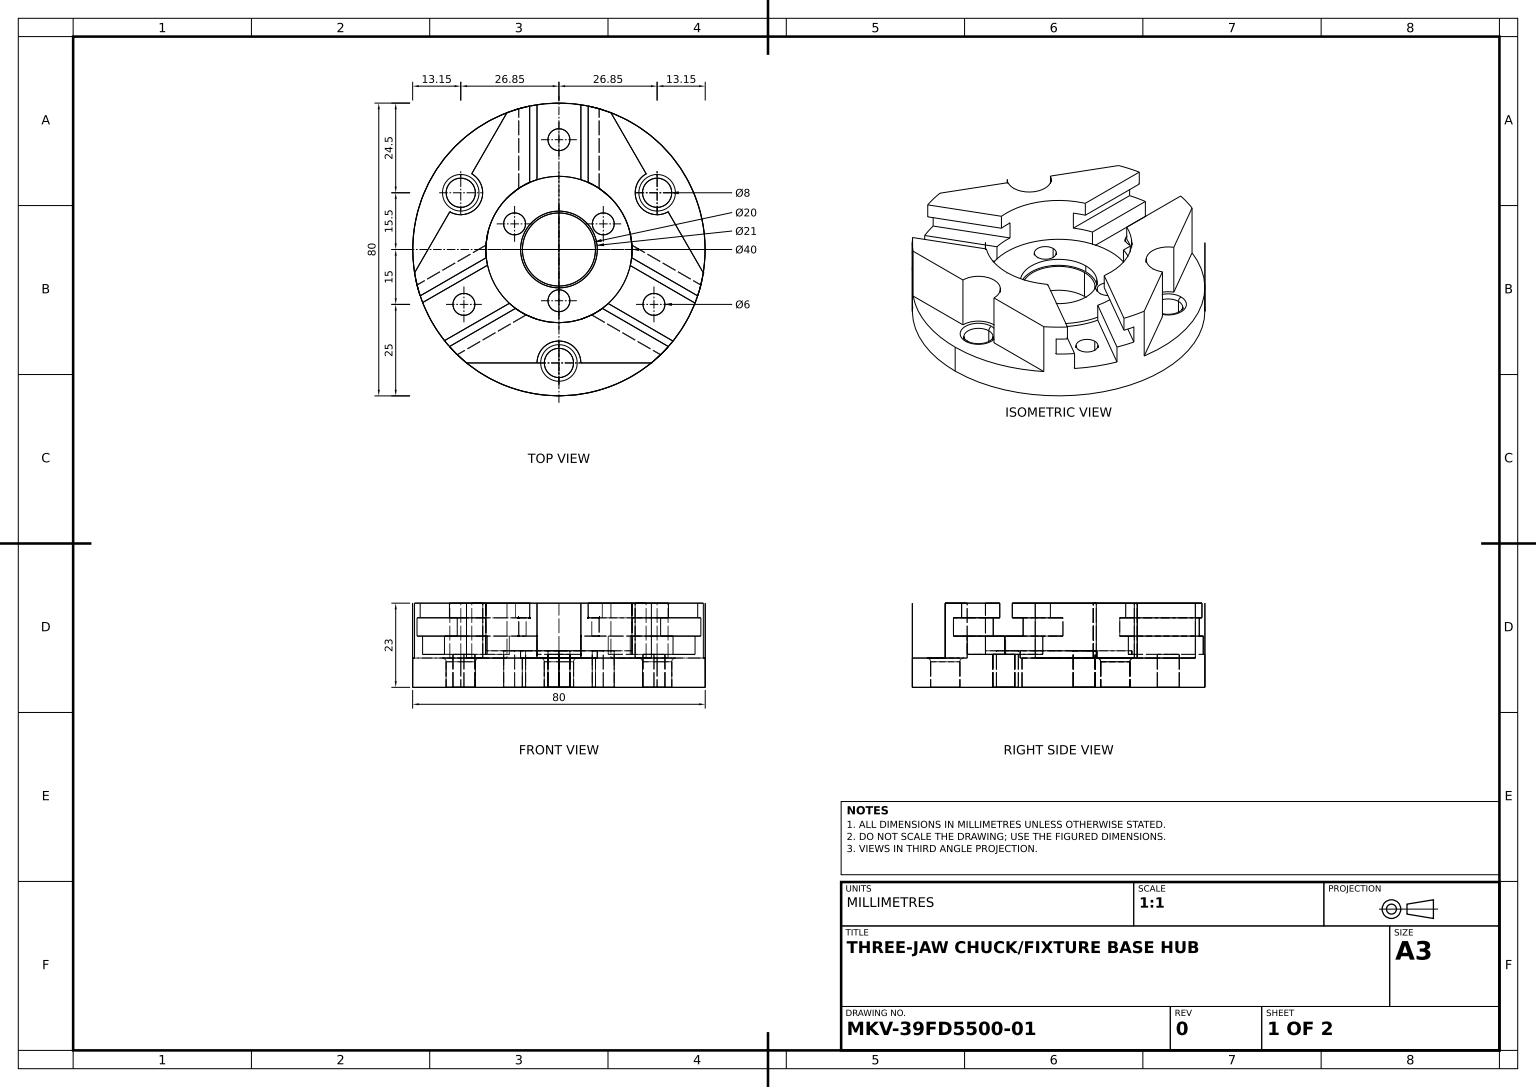
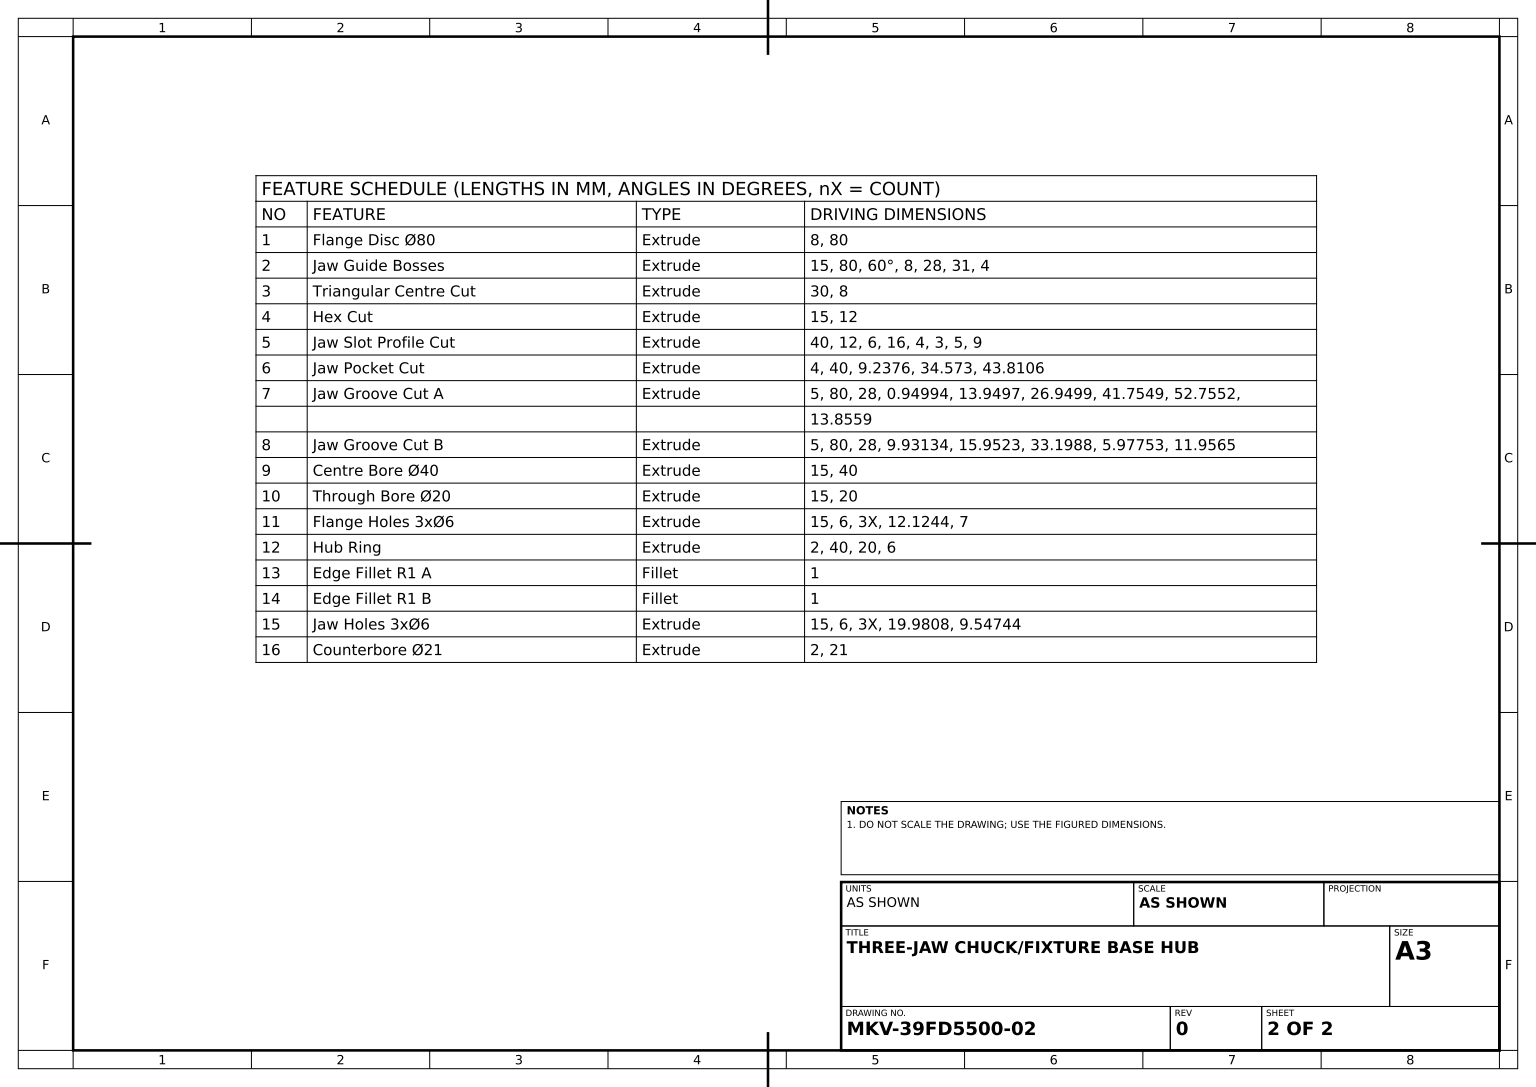
solid
v1 (25.980762,0,18)
v2 (25.980762,9,18)
e1 v1 v2 LINE
v3 (25.980762,9,12)
e2 v2 v3 CIRCLE(AX(P(25.980762,9,15),D(0,1,0),D(0,0,1)),3)
v4 (25.980762,0,12)
e3 v4 v3 LINE
e4 v1 v4 CIRCLE(AX(P(25.980762,0,15),D(0,1,0),D(0,0,1)),3)
face CYL(AX(P(25.980762,-6,15),D(0,1,0),D(0,0,1)),3) rev [e1 e2 -e3 -e4]
v5 (0,0,-10)
v6 (0,8,-10)
e5 v5 v6 LINE
v7 (0,8,10)
e6 v7 v6 CIRCLE(AX(P(0,8,0),D(0,-1,0),D(0,0,1)),10)
v8 (0,0,10)
e7 v8 v7 LINE
e8 v5 v8 CIRCLE(AX(P(0,0,0),D(0,1,0),D(0,0,1)),10)
face CYL(AX(P(0,-7,0),D(0,1,0),D(0,0,1)),10) rev [e5 -e6 -e7 -e8]
v9 (29.846788,8,-10.303848)
v10 (29.846788,23,-10.303848)
e9 v9 v10 LINE
v11 (26.846788,8,-9.5)
e10 v11 v9 CIRCLE(AX(P(26.846788,8,-15.5),D(0,1,0),D(0,0,1)),6)
v12 (26.846788,23,-9.5)
e11 v11 v12 LINE
e12 v12 v10 CIRCLE(AX(P(26.846788,23,-15.5),D(0,1,0),D(0,0,1)),6)
face CYL(AX(P(26.846788,8,-15.5),D(0,1,0),D(0,0,1)),6) rev [-e9 -e10 e11 e12]
v13 (-12.124356,0,-10)
v14 (-12.124356,0,-4)
e13 v13 v14 CIRCLE(AX(P(-12.124356,0,-7),D(0,1,0),D(0,0,1)),3)
v15 (-12.124356,10,-10)
e14 v13 v15 LINE
v16 (-12.124356,10,-4)
e15 v15 v16 CIRCLE(AX(P(-12.124356,10,-7),D(0,1,0),D(0,0,1)),3)
e16 v14 v16 LINE
face CYL(AX(P(-12.124356,-7,-7),D(0,1,0),D(0,0,1)),3) rev [-e13 e14 e15 -e16]
v17 (-8.965703,14,17.877812)
v18 (-27.80577,14,28.754811)
e17 v17 v18 LINE
v19 (-27.80577,19,28.754811)
e18 v18 v19 LINE
v20 (-8.965703,19,17.877812)
e19 v20 v19 LINE
e20 v17 v20 LINE
face PLANE(AX(P(5.499879,14,9.526349),D(-0.499989,0,-0.866031755),D(-0.866031755,0,0.499989))) [e17 e18 -e19 -e20]
v21 (-13.552446,9,14.708202)
v22 (-13.552446,10,14.708202)
e21 v21 v22 LINE
v23 (-19.531444,10,4.3038)
e22 v23 v22 CIRCLE(AX(P(0,10,0),D(0,1,0),D(0,0,1)),20)
v24 (-19.531444,9,4.3038)
e23 v24 v23 LINE
e24 v24 v21 CIRCLE(AX(P(0,9,0),D(0,1,0),D(0,0,1)),20)
face CYL(AX(P(0,10,0),D(0,-1,0),D(0,0,-1)),20) [e21 -e22 -e23 e24]
v25 (-26.846788,0,-11.5)
v26 (-26.846788,0,-19.5)
e25 v25 v26 CIRCLE(AX(P(-26.846788,0,-15.5),D(0,1,0),D(0,0,1)),4)
v27 (-26.846788,7,-11.5)
e26 v27 v25 LINE
v28 (-26.846788,7,-19.5)
e27 v27 v28 CIRCLE(AX(P(-26.846788,7,-15.5),D(0,1,0),D(0,0,1)),4)
e28 v28 v26 LINE
face CYL(AX(P(-26.846788,23,-15.5),D(0,-1,0),D(0,0,-1)),4) rev [-e25 -e26 e27 e28]
e29 v3 v2 CIRCLE(AX(P(25.980762,9,15),D(0,1,0),D(0,0,1)),3)
v29 (31.198591,9,25.032936)
v30 (37.219569,9,14.652771)
e30 v29 v30 CIRCLE(AX(P(0,9,0),D(0,1,0),D(0,0,1)),40)
v31 (19.5139,9,4.382662)
e31 v30 v31 LINE
v32 (13.492922,9,14.762827)
e32 v32 v31 CIRCLE(AX(P(0,9,0),D(0,1,0),D(0,0,1)),20)
e33 v32 v29 LINE
face PLANE(AX(P(0,9,0),D(0,1,0),D(0,0,1))) [-e2 -e29] [e30 e31 -e32 e33]
v33 (-8,19,-18.330303)
v34 (-8,19,-39.191836)
e34 v33 v34 LINE
v35 (-11,19,-16.703293)
e35 v35 v33 CIRCLE(AX(P(0,19,0),D(0,-1,0),D(0,0,-1)),20)
v36 (-11,19,-38.457769)
e36 v35 v36 LINE
e37 v36 v34 CIRCLE(AX(P(0,19,0),D(0,-1,0),D(0,0,-1)),40)
face PLANE(AX(P(-8,19,0),D(0,-1,0),D(0,0,-1))) [-e34 -e35 e36 e37]
v37 (8,23,-18.330303)
v38 (8,19,-18.330303)
e38 v37 v38 LINE
v39 (11,19,-16.703293)
e39 v38 v39 CIRCLE(AX(P(0,19,0),D(0,-1,0),D(0,0,-1)),20)
v40 (11,14,-16.703293)
e40 v39 v40 LINE
v41 (6,14,-19.078784)
e41 v40 v41 CIRCLE(AX(P(0,14,0),D(0,1,0),D(-1,0,0)),20)
v42 (6,10,-19.078784)
e42 v41 v42 LINE
v43 (19.5139,10,4.382662)
e43 v43 v42 CIRCLE(AX(P(0,10,0),D(0,1,0),D(0,0,1)),20)
v44 (19.5139,14,4.382662)
e44 v44 v43 LINE
v45 (19.965491,14,-1.174379)
e45 v44 v45 CIRCLE(AX(P(0,14,0),D(0,1,0),D(0,0,1)),20)
v46 (19.965491,19,-1.174379)
e46 v45 v46 LINE
v47 (19.874508,19,2.236948)
e47 v47 v46 CIRCLE(AX(P(0,19,0),D(0,1,0),D(0,0,1)),20)
v48 (19.874508,23,2.236948)
e48 v48 v47 LINE
e49 v48 v37 CIRCLE(AX(P(0,23,0),D(0,1,0),D(0,0,1)),20)
face CYL(AX(P(0,8,0),D(0,1,0),D(0,0,1)),20) rev [e38 e39 e40 e41 e42 -e43 -e44 e45 e46 -e47 -e48 e49]
v49 (13.492922,10,14.762827)
v50 (13.492922,14,14.762827)
e50 v49 v50 LINE
v51 (31.198591,14,25.032936)
e51 v50 v51 LINE
e52 v29 v51 LINE
e53 v32 v49 LINE
face PLANE(AX(P(7.931166,9,11.53675),D(-0.501748125,0,0.865013768),D(0.865013768,0,0.501748125))) rev [e50 e51 -e52 -e33 e53]
v52 (-37.278454,9,14.502304)
e54 v24 v52 LINE
v53 (-31.299456,9,24.906706)
e55 v52 v53 CIRCLE(AX(P(0,9,0),D(0,1,0),D(0,0,1)),40)
e56 v53 v21 LINE
v54 (-25.980762,9,18)
v55 (-25.980762,9,12)
e57 v54 v55 CIRCLE(AX(P(-25.980762,9,15),D(0,1,0),D(0,0,1)),3)
e58 v55 v54 CIRCLE(AX(P(-25.980762,9,15),D(0,1,0),D(0,0,1)),3)
face PLANE(AX(P(0,9,0),D(0,1,0),D(0,0,1))) [-e24 e54 e55 e56] [-e57 -e58]
v56 (14.207563,23,-37.391779)
v57 (8,23,-39.191836)
e59 v56 v57 CIRCLE(AX(P(0,23,0),D(0,1,0),D(0,0,1)),40)
v58 (14.207563,8,-37.391779)
e60 v56 v58 LINE
v59 (39.486012,8,6.391779)
e61 v59 v58 CIRCLE(AX(P(0,8,0),D(0,1,0),D(0,0,1)),40)
v60 (39.486012,23,6.391779)
e62 v60 v59 LINE
v61 (37.941125,23,12.667715)
e63 v61 v60 CIRCLE(AX(P(0,23,0),D(0,1,0),D(0,0,1)),40)
v62 (37.941125,19,12.667715)
e64 v62 v61 LINE
v63 (38.805282,19,9.703098)
e65 v62 v63 CIRCLE(AX(P(0,19,0),D(0,1,0),D(0,0,1)),40)
v64 (38.805282,14,9.703098)
e66 v64 v63 LINE
v65 (37.219569,14,14.652771)
e67 v65 v64 CIRCLE(AX(P(0,14,0),D(0,1,0),D(0,0,1)),40)
e68 v30 v65 LINE
v66 (27.80504,14,28.755517)
e69 v66 v51 CIRCLE(AX(P(0,14,0),D(0,1,0),D(0,0,1)),40)
v67 (27.80504,19,28.755517)
e70 v66 v67 LINE
v68 (29.941125,19,26.524121)
e71 v67 v68 CIRCLE(AX(P(0,19,0),D(0,1,0),D(0,0,1)),40)
v69 (29.941125,23,26.524121)
e72 v68 v69 LINE
v70 (25.278449,23,31)
e73 v70 v69 CIRCLE(AX(P(0,23,0),D(0,1,0),D(0,0,1)),40)
v71 (25.278449,8,31)
e74 v70 v71 LINE
v72 (0,8,40)
e75 v72 v71 CIRCLE(AX(P(0,8,0),D(0,1,0),D(0,0,1)),40)
v73 (0,0,40)
e76 v72 v73 LINE
v74 (0,0,-40)
e77 v73 v74 CIRCLE(AX(P(0,0,0),D(0,1,0),D(0,0,1)),40)
v75 (0,9,-40)
e78 v75 v74 LINE
v76 (6,9,-39.54744)
e79 v76 v75 CIRCLE(AX(P(0,9,0),D(0,1,0),D(0,0,1)),40)
v77 (6,14,-39.54744)
e80 v77 v76 LINE
v78 (11,14,-38.457769)
e81 v78 v77 CIRCLE(AX(P(0,14,0),D(0,1,0),D(-1,0,0)),40)
v79 (11,19,-38.457769)
e82 v79 v78 LINE
v80 (8,19,-39.191836)
e83 v80 v79 CIRCLE(AX(P(0,19,0),D(0,-1,0),D(0,0,-1)),40)
e84 v57 v80 LINE
face CYL(AX(P(0,8,0),D(0,-1,0),D(0,0,-1)),40) [-e59 e60 -e61 -e62 -e63 -e64 e65 -e66 -e67 -e68 -e30 e52 -e69 e70 e71 e72 -e73 e74 -e75 e76 e77 -e78 -e79 -e80 -e81 -e82 -e83 -e84]
v81 (-25.980762,0,12)
e85 v81 v55 LINE
v82 (-25.980762,0,18)
e86 v82 v81 CIRCLE(AX(P(-25.980762,0,15),D(0,1,0),D(0,0,1)),3)
e87 v82 v54 LINE
face CYL(AX(P(-25.980762,-6,15),D(0,1,0),D(0,0,1)),3) rev [e57 -e85 -e86 e87]
v83 (12.124356,0,-4)
v84 (12.124356,0,-10)
e88 v83 v84 CIRCLE(AX(P(12.124356,0,-7),D(0,1,0),D(0,0,1)),3)
v85 (12.124356,10,-4)
e89 v83 v85 LINE
v86 (12.124356,10,-10)
e90 v85 v86 CIRCLE(AX(P(12.124356,10,-7),D(0,1,0),D(0,0,1)),3)
e91 v84 v86 LINE
face CYL(AX(P(12.124356,-7,-7),D(0,1,0),D(0,0,1)),3) rev [-e88 e89 e90 -e91]
v87 (-8,23,-18.330303)
e92 v33 v87 LINE
v88 (-19.874508,23,2.236948)
e93 v87 v88 CIRCLE(AX(P(0,23,0),D(0,1,0),D(0,0,1)),20)
v89 (-19.874508,19,2.236948)
e94 v89 v88 LINE
v90 (-19.965461,19,-1.174887)
e95 v90 v89 CIRCLE(AX(P(0,19,0),D(0,1,0),D(0,0,1)),20)
v91 (-19.965461,14,-1.174887)
e96 v91 v90 LINE
v92 (-19.531444,14,4.3038)
e97 v91 v92 CIRCLE(AX(P(0,14,0),D(0,1,0),D(0,0,1)),20)
e98 v23 v92 LINE
v93 (-6,10,-19.078784)
e99 v93 v23 CIRCLE(AX(P(0,10,0),D(0,1,0),D(0,0,1)),20)
v94 (-6,14,-19.078784)
e100 v93 v94 LINE
v95 (-11,14,-16.703293)
e101 v94 v95 CIRCLE(AX(P(0,14,0),D(0,1,0),D(0,0,1)),20)
e102 v95 v35 LINE
face CYL(AX(P(0,8,0),D(0,1,0),D(0,0,1)),20) rev [e92 e93 -e94 -e95 -e96 e97 -e98 -e99 e100 e101 e102 e35]
v96 (26.846788,0,-19.5)
v97 (26.846788,0,-11.5)
e103 v96 v97 CIRCLE(AX(P(26.846788,0,-15.5),D(0,1,0),D(0,0,1)),4)
v98 (26.846788,7,-19.5)
e104 v98 v96 LINE
v99 (26.846788,7,-11.5)
e105 v98 v99 CIRCLE(AX(P(26.846788,7,-15.5),D(0,1,0),D(0,0,1)),4)
e106 v99 v97 LINE
face CYL(AX(P(26.846788,23,-15.5),D(0,-1,0),D(0,0,-1)),4) rev [-e103 -e104 e105 e106]
v100 (-6,9,-39.54744)
e107 v75 v100 CIRCLE(AX(P(0,9,0),D(0,1,0),D(0,0,1)),40)
e108 v74 v73 CIRCLE(AX(P(0,0,0),D(0,1,0),D(0,0,1)),40)
v101 (-25.278449,8,31)
e109 v101 v72 CIRCLE(AX(P(0,8,0),D(0,1,0),D(0,0,1)),40)
v102 (-25.278449,23,31)
e110 v102 v101 LINE
v103 (-29.941125,23,26.524121)
e111 v103 v102 CIRCLE(AX(P(0,23,0),D(0,1,0),D(0,0,1)),40)
v104 (-29.941125,19,26.524121)
e112 v104 v103 LINE
e113 v104 v19 CIRCLE(AX(P(0,19,0),D(0,1,0),D(0,0,1)),40)
v105 (-31.299456,14,24.906706)
e114 v105 v18 CIRCLE(AX(P(0,14,0),D(0,1,0),D(0,0,1)),40)
e115 v53 v105 LINE
v106 (-37.278454,14,14.502304)
e116 v52 v106 LINE
v107 (-38.805528,14,9.702112)
e117 v107 v106 CIRCLE(AX(P(0,14,0),D(0,1,0),D(0,0,1)),40)
v108 (-38.805528,19,9.702112)
e118 v107 v108 LINE
v109 (-37.941125,19,12.667715)
e119 v108 v109 CIRCLE(AX(P(0,19,0),D(0,1,0),D(0,0,1)),40)
v110 (-37.941125,23,12.667715)
e120 v109 v110 LINE
v111 (-39.486012,23,6.391779)
e121 v111 v110 CIRCLE(AX(P(0,23,0),D(0,1,0),D(0,0,1)),40)
v112 (-39.486012,8,6.391779)
e122 v111 v112 LINE
v113 (-14.207563,8,-37.391779)
e123 v113 v112 CIRCLE(AX(P(0,8,0),D(0,1,0),D(0,0,1)),40)
v114 (-14.207563,23,-37.391779)
e124 v114 v113 LINE
v115 (-8,23,-39.191836)
e125 v115 v114 CIRCLE(AX(P(0,23,0),D(0,1,0),D(0,0,1)),40)
e126 v34 v115 LINE
v116 (-11,14,-38.457769)
e127 v116 v36 LINE
v117 (-6,14,-39.54744)
e128 v117 v116 CIRCLE(AX(P(0,14,0),D(0,1,0),D(0,0,1)),40)
e129 v100 v117 LINE
face CYL(AX(P(0,8,0),D(0,-1,0),D(0,0,-1)),40) [-e107 e78 e108 -e76 -e109 -e110 -e111 -e112 e113 -e18 -e114 -e115 -e55 e116 -e117 e118 e119 e120 -e121 e122 -e123 -e124 -e125 -e126 -e37 -e127 -e128 -e129]
e130 v87 v115 LINE
v118 (-23.846788,23,-20.696152)
e131 v114 v118 LINE
v119 (-26.846788,23,-9.5)
e132 v119 v118 CIRCLE(AX(P(-26.846788,23,-15.5),D(0,1,0),D(0,0,1)),6)
v120 (-29.846788,23,-10.303848)
e133 v120 v119 CIRCLE(AX(P(-26.846788,23,-15.5),D(0,1,0),D(0,0,1)),6)
e134 v120 v111 LINE
e135 v88 v110 LINE
face PLANE(AX(P(0,23,0),D(0,1,0),D(0,0,1))) [e130 e125 e131 -e132 -e133 e134 e121 -e135 -e93]
e136 v39 v79 LINE
e137 v40 v78 LINE
face PLANE(AX(P(11,19,0),D(-1,0,0),D(0,-1,0))) [e136 e82 -e137 -e40]
v121 (6,8,31)
v122 (-6,8,31)
e138 v121 v122 CIRCLE(AX(P(0,8,31),D(0,1,0),D(0,0,1)),6)
e139 v122 v101 LINE
e140 v71 v121 LINE
v123 (0,8,36)
v124 (0,8,26)
e141 v123 v124 CIRCLE(AX(P(0,8,31),D(0,-1,0),D(0,0,1)),5)
e142 v124 v123 CIRCLE(AX(P(0,8,31),D(0,-1,0),D(0,0,1)),5)
face PLANE(AX(P(0,8,0),D(0,1,0),D(0,0,1))) [e138 e139 e109 e75 e140] [e141 e142]
v125 (0,9,-27)
v126 (0,9,-33)
e143 v125 v126 CIRCLE(AX(P(0,9,-30),D(0,1,0),D(0,0,1)),3)
v127 (0,0,-33)
e144 v127 v126 LINE
v128 (0,0,-27)
e145 v128 v127 CIRCLE(AX(P(0,0,-30),D(0,1,0),D(0,0,1)),3)
e146 v128 v125 LINE
face CYL(AX(P(0,-6,-30),D(0,1,0),D(0,0,1)),3) rev [e143 -e144 -e145 e146]
e147 v38 v80 LINE
e148 v57 v37 LINE
face PLANE(AX(P(8,23,0),D(-1,0,0),D(0,0,1))) [-e147 -e38 -e148 e84]
e149 v126 v125 CIRCLE(AX(P(0,9,-30),D(0,1,0),D(0,0,1)),3)
v129 (6,9,-19.078784)
v130 (0,9,-20)
e150 v129 v130 CIRCLE(AX(P(0,9,0),D(0,1,0),D(0,0,1)),20)
e151 v129 v76 LINE
v131 (-6,9,-19.078784)
e152 v131 v100 LINE
e153 v130 v131 CIRCLE(AX(P(0,9,0),D(0,1,0),D(0,0,1)),20)
face PLANE(AX(P(-6,9,0),D(0,1,0),D(0,0,1))) [-e149 -e143] [-e150 e151 e79 e107 -e152 -e153]
v132 (-13.552446,14,14.708202)
e154 v105 v132 LINE
e155 v132 v22 LINE
face PLANE(AX(P(-7.977704,9,11.504618),D(0.498249835,0,0.867033507),D(0.867033507,0,-0.498249835))) rev [e154 e155 -e21 -e56 e115]
v133 (11.874508,19,16.093355)
e156 v133 v68 LINE
v134 (11.874508,23,16.093355)
e157 v133 v134 LINE
e158 v134 v69 LINE
face PLANE(AX(P(0,19,9.237604),D(-0.5,0,0.866025404),D(0.866025404,0,0.5))) rev [-e72 -e156 e157 e158]
v135 (-29.846788,8,-10.303848)
e159 v135 v120 LINE
e160 v135 v112 LINE
face PLANE(AX(P(-26.846788,23,-15.5),D(0.866025404,0,0.5),D(0.5,0,-0.866025404))) rev [-e122 -e134 -e159 e160]
e161 v131 v93 LINE
v136 (0,10,-20)
e162 v136 v93 CIRCLE(AX(P(0,10,0),D(0,1,0),D(0,0,1)),20)
e163 v136 v130 LINE
face CYL(AX(P(0,10,0),D(0,-1,0),D(0,0,-1)),20) [e161 -e162 e163 e153]
e164 v81 v82 CIRCLE(AX(P(-25.980762,0,15),D(0,1,0),D(0,0,1)),3)
face CYL(AX(P(-25.980762,-6,15),D(0,1,0),D(0,0,1)),3) rev [e58 -e87 -e164 e85]
v137 (26.846788,8,-20.5)
e165 v137 v98 CIRCLE(AX(P(26.846788,7,-20.5),D(1,0,0),D(0,0,-1)),1)
e166 v99 v98 CIRCLE(AX(P(26.846788,7,-15.5),D(0,1,0),D(0,0,1)),4)
v138 (26.846788,8,-10.5)
e167 v138 v99 CIRCLE(AX(P(26.846788,7,-10.5),D(-1,0,0),D(0,0,1)),1)
e168 v137 v138 CIRCLE(AX(P(26.846788,8,-15.5),D(0,-1,0),D(0,0,1)),5)
face TORUS(AX(P(26.846788,7,-15.5),D(0,1,0),D(0,0,1)),5,1) [e165 -e166 -e167 -e168]
e169 v127 v128 CIRCLE(AX(P(0,0,-30),D(0,1,0),D(0,0,1)),3)
face CYL(AX(P(0,-6,-30),D(0,1,0),D(0,0,1)),3) rev [e149 -e146 -e169 e144]
e170 v4 v1 CIRCLE(AX(P(25.980762,0,15),D(0,1,0),D(0,0,1)),3)
face CYL(AX(P(25.980762,-6,15),D(0,1,0),D(0,0,1)),3) rev [-e1 -e170 e3 e29]
v139 (0,7,35)
v140 (0,0,35)
e171 v139 v140 LINE
v141 (0,0,27)
e172 v141 v140 CIRCLE(AX(P(0,0,31),D(0,1,0),D(0,0,1)),4)
v142 (0,7,27)
e173 v142 v141 LINE
e174 v142 v139 CIRCLE(AX(P(0,7,31),D(0,1,0),D(0,0,1)),4)
face CYL(AX(P(0,23,31),D(0,-1,0),D(0,0,-1)),4) rev [e171 -e172 -e173 e174]
v143 (0,10,20)
e175 v143 v49 CIRCLE(AX(P(0,10,0),D(0,1,0),D(0,0,1)),20)
v144 (0,23,20)
e176 v143 v144 LINE
e177 v144 v134 CIRCLE(AX(P(0,23,0),D(0,1,0),D(0,0,1)),20)
v145 (8.965249,19,17.87804)
e178 v145 v133 CIRCLE(AX(P(0,19,0),D(0,1,0),D(0,0,1)),20)
v146 (8.965249,14,17.87804)
e179 v146 v145 LINE
e180 v146 v50 CIRCLE(AX(P(0,14,0),D(0,1,0),D(0,0,1)),20)
face CYL(AX(P(0,8,0),D(0,1,0),D(0,0,1)),20) rev [-e50 -e175 e176 e177 -e157 -e178 -e179 e180]
e181 v124 v142 CIRCLE(AX(P(0,7,26),D(1,0,0),D(0,0,-1)),1)
e182 v123 v139 CIRCLE(AX(P(0,7,36),D(-1,0,0),D(0,0,1)),1)
face TORUS(AX(P(0,7,31),D(0,1,0),D(0,0,1)),5,1) [-e174 -e181 -e141 e182]
v147 (0,8,10.5)
v148 (0,8,-10.5)
e183 v147 v148 CIRCLE(AX(P(0,8,0),D(0,1,0),D(0,0,1)),10.5)
e184 v148 v147 CIRCLE(AX(P(0,8,0),D(0,1,0),D(0,0,1)),10.5)
e185 v6 v7 CIRCLE(AX(P(0,8,0),D(0,-1,0),D(0,0,1)),10)
face PLANE(AX(P(0,8,0),D(0,1,0),D(0,0,1))) [e183 e184] [e185 e6]
e186 v145 v67 LINE
face PLANE(AX(P(0,19,0),D(0,1,0),D(0,0,1))) rev [e156 -e71 -e186 e178]
e187 v84 v83 CIRCLE(AX(P(12.124356,0,-7),D(0,1,0),D(0,0,1)),3)
e188 v86 v85 CIRCLE(AX(P(12.124356,10,-7),D(0,1,0),D(0,0,1)),3)
face CYL(AX(P(12.124356,-7,-7),D(0,1,0),D(0,0,1)),3) rev [-e89 -e187 e91 e188]
e189 v132 v17 CIRCLE(AX(P(0,14,0),D(0,1,0),D(0,0,1)),20)
face PLANE(AX(P(0,14,0),D(0,1,0),D(0,0,1))) [e114 -e17 -e189 -e154]
v149 (-11.874508,19,16.093355)
e190 v149 v20 CIRCLE(AX(P(0,19,0),D(0,1,0),D(0,0,1)),20)
v150 (-11.874508,23,16.093355)
e191 v150 v149 LINE
e192 v150 v144 CIRCLE(AX(P(0,23,0),D(0,1,0),D(0,0,1)),20)
e193 v22 v143 CIRCLE(AX(P(0,10,0),D(0,1,0),D(0,0,1)),20)
face CYL(AX(P(0,8,0),D(0,1,0),D(0,0,1)),20) rev [-e155 e189 e20 -e190 -e191 e192 -e176 -e193]
e194 v89 v109 LINE
face PLANE(AX(P(0,19,-9.237604),D(-0.5,0,-0.866025404),D(-0.866025404,0,0.5))) rev [e94 e135 -e120 -e194]
e195 v94 v117 LINE
face PLANE(AX(P(-6,14,0),D(1,0,0),D(0,1,0))) [e129 -e195 -e100 -e161 e152]
v151 (-23.846788,8,-20.696152)
e196 v151 v118 LINE
v152 (-26.846788,8,-9.5)
e197 v152 v151 CIRCLE(AX(P(-26.846788,8,-15.5),D(0,1,0),D(0,0,1)),6)
e198 v152 v119 LINE
face CYL(AX(P(-26.846788,8,-15.5),D(0,1,0),D(0,0,1)),6) rev [-e196 -e197 e198 e132]
v153 (23.846788,8,-20.696152)
e199 v58 v153 LINE
v154 (23.846788,23,-20.696152)
e200 v56 v154 LINE
e201 v153 v154 LINE
face PLANE(AX(P(26.846788,23,-15.5),D(0.866025404,0,-0.5),D(-0.5,0,-0.866025404))) [-e199 -e60 e200 -e201]
e202 v91 v107 LINE
e203 v92 v106 LINE
face PLANE(AX(P(0,14,0),D(0,1,0),D(0,0,1))) [-e97 e202 e117 -e203]
v155 (0,10,11)
v156 (0,10,17)
e204 v155 v156 CIRCLE(AX(P(0,10,14),D(0,1,0),D(0,0,1)),3)
v157 (0,0,17)
e205 v157 v156 LINE
v158 (0,0,11)
e206 v158 v157 CIRCLE(AX(P(0,0,14),D(0,1,0),D(0,0,1)),3)
e207 v158 v155 LINE
face CYL(AX(P(0,-7,14),D(0,1,0),D(0,0,1)),3) rev [e204 -e205 -e206 e207]
e208 v104 v149 LINE
face PLANE(AX(P(0,19,0),D(0,1,0),D(0,0,1))) rev [-e113 e208 e190 e19]
v159 (6,23,31)
e209 v70 v159 LINE
e210 v121 v159 LINE
face PLANE(AX(P(0,23,31),D(0,0,1),D(1,0,0))) [-e74 e209 -e210 -e140]
e211 v129 v42 LINE
e212 v41 v77 LINE
face PLANE(AX(P(6,14,0),D(-1,0,0),D(0,-1,0))) [e80 -e151 e211 -e42 e212]
e213 v49 v43 CIRCLE(AX(P(0,10,0),D(0,1,0),D(0,0,1)),20)
e214 v42 v136 CIRCLE(AX(P(0,10,0),D(0,1,0),D(0,0,1)),20)
e215 v16 v15 CIRCLE(AX(P(-12.124356,10,-7),D(0,1,0),D(0,0,1)),3)
v160 (0,10,10.5)
v161 (0,10,-10.5)
e216 v160 v161 CIRCLE(AX(P(0,10,0),D(0,1,0),D(0,0,1)),10.5)
e217 v161 v160 CIRCLE(AX(P(0,10,0),D(0,1,0),D(0,0,1)),10.5)
e218 v156 v155 CIRCLE(AX(P(0,10,14),D(0,1,0),D(0,0,1)),3)
face PLANE(AX(P(0,10,0),D(0,1,0),D(0,0,1))) [e22 e193 e175 e213 e43 e214 e162 e99] [-e15 -e215] [-e90 -e188] [-e216 -e217] [-e218 -e204]
e219 v113 v151 LINE
face PLANE(AX(P(-26.846788,23,-15.5),D(0.866025404,0,0.5),D(0.5,0,-0.866025404))) rev [e196 -e131 e124 e219]
e220 v135 v152 CIRCLE(AX(P(-26.846788,8,-15.5),D(0,1,0),D(0,0,1)),6)
v162 (-26.846788,8,-20.5)
v163 (-26.846788,8,-10.5)
e221 v162 v163 CIRCLE(AX(P(-26.846788,8,-15.5),D(0,-1,0),D(0,0,1)),5)
e222 v163 v162 CIRCLE(AX(P(-26.846788,8,-15.5),D(0,-1,0),D(0,0,1)),5)
face PLANE(AX(P(0,8,0),D(0,1,0),D(0,0,1))) [e197 -e219 e123 -e160 e220] [e221 e222]
face CYL(AX(P(0,10,0),D(0,-1,0),D(0,0,-1)),20) [-e163 -e214 -e211 e150]
e223 v103 v150 LINE
face PLANE(AX(P(0,19,9.237604),D(0.5,0,0.866025404),D(0.866025404,0,-0.5))) rev [e112 e223 e191 -e208]
e224 v139 v142 CIRCLE(AX(P(0,7,31),D(0,1,0),D(0,0,1)),4)
face TORUS(AX(P(0,7,31),D(0,1,0),D(0,0,1)),5,1) [-e224 -e182 -e142 e181]
face PLANE(AX(P(-8,23,0),D(1,0,0),D(0,0,-1))) [-e130 -e92 e34 e126]
e225 v138 v137 CIRCLE(AX(P(26.846788,8,-15.5),D(0,-1,0),D(0,0,1)),5)
face TORUS(AX(P(26.846788,7,-15.5),D(0,1,0),D(0,0,1)),5,1) [-e165 -e225 e167 -e105]
face PLANE(AX(P(11,14,0),D(0,1,0),D(-1,0,0))) [-e212 -e41 e137 e81]
v164 (-6,23,31)
e226 v164 v102 LINE
e227 v159 v164 CIRCLE(AX(P(0,23,31),D(0,1,0),D(0,0,1)),6)
face PLANE(AX(P(0,23,0),D(0,1,0),D(0,0,1))) [-e226 -e227 -e209 e73 -e158 -e177 -e192 -e223 e111]
e228 v122 v164 LINE
face PLANE(AX(P(0,23,31),D(0,0,1),D(1,0,0))) [e228 e226 e110 -e139]
e229 v8 v5 CIRCLE(AX(P(0,0,0),D(0,1,0),D(0,0,1)),10)
face CYL(AX(P(0,-7,0),D(0,1,0),D(0,0,1)),10) rev [-e229 e7 -e185 -e5]
e230 v90 v108 LINE
face PLANE(AX(P(0,19,0),D(0,1,0),D(0,0,1))) rev [-e119 -e230 e95 e194]
e231 v146 v66 LINE
face PLANE(AX(P(-5.500121,14,9.52621),D(-0.500011,0,0.866019053),D(0.866019053,0,0.500011))) rev [e179 e186 -e70 -e231]
face CYL(AX(P(-26.846788,8,-15.5),D(0,1,0),D(0,0,1)),6) rev [e133 -e198 -e220 e159]
e232 v97 v96 CIRCLE(AX(P(26.846788,0,-15.5),D(0,1,0),D(0,0,1)),4)
face CYL(AX(P(26.846788,23,-15.5),D(0,-1,0),D(0,0,-1)),4) rev [-e232 -e106 e166 e104]
e233 v95 v116 LINE
face PLANE(AX(P(-11,14,0),D(0,1,0),D(0,0,1))) [-e233 -e101 e195 e128]
face PLANE(AX(P(-13.956702,9,1.100216),D(-0.498249835,0,-0.867033507),D(-0.867033507,0,0.498249835))) rev [-e116 -e54 e23 e98 e203]
e234 v153 v11 CIRCLE(AX(P(26.846788,8,-15.5),D(0,1,0),D(0,0,1)),6)
e235 v9 v59 LINE
face PLANE(AX(P(0,8,0),D(0,1,0),D(0,0,1))) [e168 e225] [e234 e10 e235 e61 e199]
e236 v162 v28 CIRCLE(AX(P(-26.846788,7,-20.5),D(1,0,0),D(0,0,-1)),1)
e237 v163 v27 CIRCLE(AX(P(-26.846788,7,-10.5),D(-1,0,0),D(0,0,1)),1)
face TORUS(AX(P(-26.846788,7,-15.5),D(0,1,0),D(0,0,1)),5,1) [e236 -e27 -e237 -e221]
e238 v140 v141 CIRCLE(AX(P(0,0,31),D(0,1,0),D(0,0,1)),4)
face CYL(AX(P(0,23,31),D(0,-1,0),D(0,0,-1)),4) rev [e224 e173 -e238 -e171]
e239 v46 v63 LINE
e240 v62 v47 LINE
face PLANE(AX(P(0,19,0),D(0,1,0),D(0,0,1))) rev [e47 e239 -e65 e240]
e241 v154 v12 CIRCLE(AX(P(26.846788,23,-15.5),D(0,1,0),D(0,0,1)),6)
face CYL(AX(P(26.846788,8,-15.5),D(0,1,0),D(0,0,1)),6) rev [e241 -e11 -e234 e201]
e242 v14 v13 CIRCLE(AX(P(-12.124356,0,-7),D(0,1,0),D(0,0,1)),3)
face CYL(AX(P(-12.124356,-7,-7),D(0,1,0),D(0,0,1)),3) rev [-e14 -e242 e16 e215]
e243 v61 v48 LINE
face PLANE(AX(P(0,19,-9.237604),D(0.5,0,-0.866025404),D(-0.866025404,0,-0.5))) rev [e64 e243 e48 -e240]
e244 v157 v158 CIRCLE(AX(P(0,0,14),D(0,1,0),D(0,0,1)),3)
face CYL(AX(P(0,-7,14),D(0,1,0),D(0,0,1)),3) rev [-e207 -e244 e205 e218]
face PLANE(AX(P(0,14,0),D(0,1,0),D(0,0,1))) [e231 e69 -e51 -e180]
e245 v31 v43 LINE
face CYL(AX(P(0,10,0),D(0,-1,0),D(0,0,-1)),20) [e32 e245 -e213 -e53]
e246 v45 v64 LINE
face PLANE(AX(P(5.500121,14,-9.52621),D(-0.500011,0,0.866019053),D(0.866019053,0,0.500011))) [e66 -e239 -e46 e246]
e247 v10 v60 LINE
face PLANE(AX(P(26.846788,23,-15.5),D(0.866025404,0,-0.5),D(-0.5,0,-0.866025404))) [e247 e62 -e235 e9]
face PLANE(AX(P(-5.499879,14,-9.526349),D(-0.499989,0,-0.866031755),D(-0.866031755,0,0.499989))) rev [e230 -e118 -e202 e96]
e248 v65 v44 LINE
face PLANE(AX(P(0,14,0),D(0,1,0),D(0,0,1))) [e67 -e246 -e45 -e248]
e249 v147 v160 LINE
e250 v148 v161 LINE
face CYL(AX(P(0,8,0),D(0,1,0),D(0,0,1)),10.5) rev [-e183 e249 e216 -e250]
e251 v28 v27 CIRCLE(AX(P(-26.846788,7,-15.5),D(0,1,0),D(0,0,1)),4)
face TORUS(AX(P(-26.846788,7,-15.5),D(0,1,0),D(0,0,1)),5,1) [-e251 -e236 -e222 e237]
face PLANE(AX(P(13.952144,9,1.156585),D(0.501748125,0,-0.865013768),D(-0.865013768,0,-0.501748125))) rev [e44 -e245 -e31 e68 e248]
face PLANE(AX(P(-11,19,0),D(1,0,0),D(0,1,0))) [-e102 e233 e127 -e36]
e252 v26 v25 CIRCLE(AX(P(-26.846788,0,-15.5),D(0,1,0),D(0,0,1)),4)
face PLANE(AX(P(0,0,0),D(0,1,0),D(0,0,1))) rev [e164 e86] [e206 e244] [e170 e4] [e103 e232] [e252 e25] [e187 e88] [e8 e229] [e172 e238] [-e108 -e77] [e13 e242] [e145 e169]
face CYL(AX(P(-26.846788,23,-15.5),D(0,-1,0),D(0,0,-1)),4) rev [e26 -e252 -e28 e251]
face CYL(AX(P(0,8,0),D(0,1,0),D(0,0,1)),10.5) rev [-e249 -e184 e250 e217]
face PLANE(AX(P(8,19,0),D(0,-1,0),D(0,0,-1))) [-e39 e147 e83 -e136]
face CYL(AX(P(0,8,31),D(0,1,0),D(0,0,1)),6) rev [e210 e227 -e228 -e138]
face PLANE(AX(P(0,23,0),D(0,1,0),D(0,0,1))) [e63 -e247 -e12 -e241 -e200 e59 e148 -e49 -e243]
